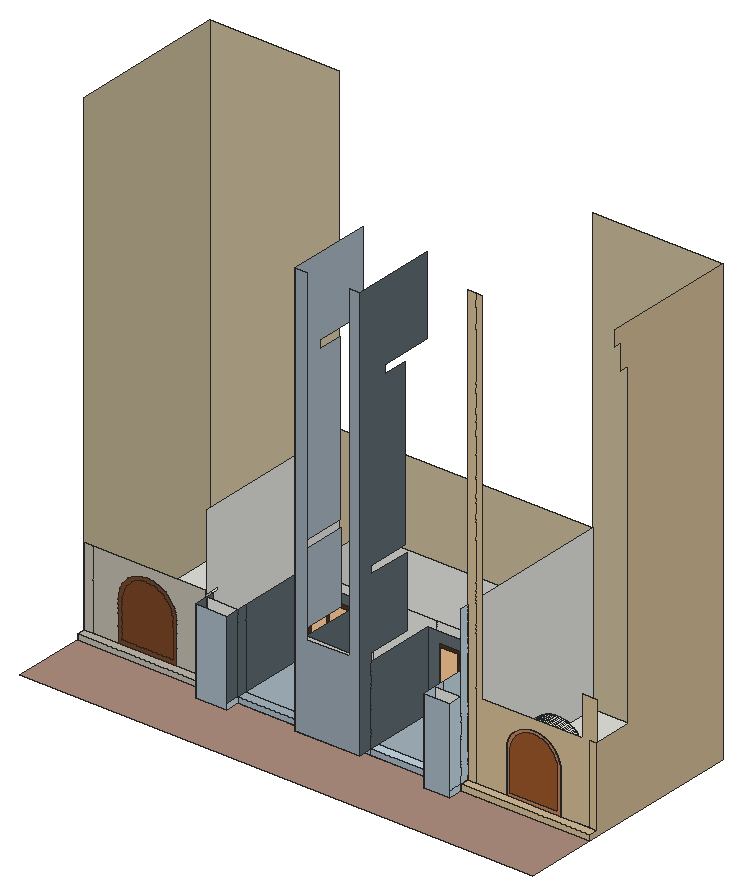
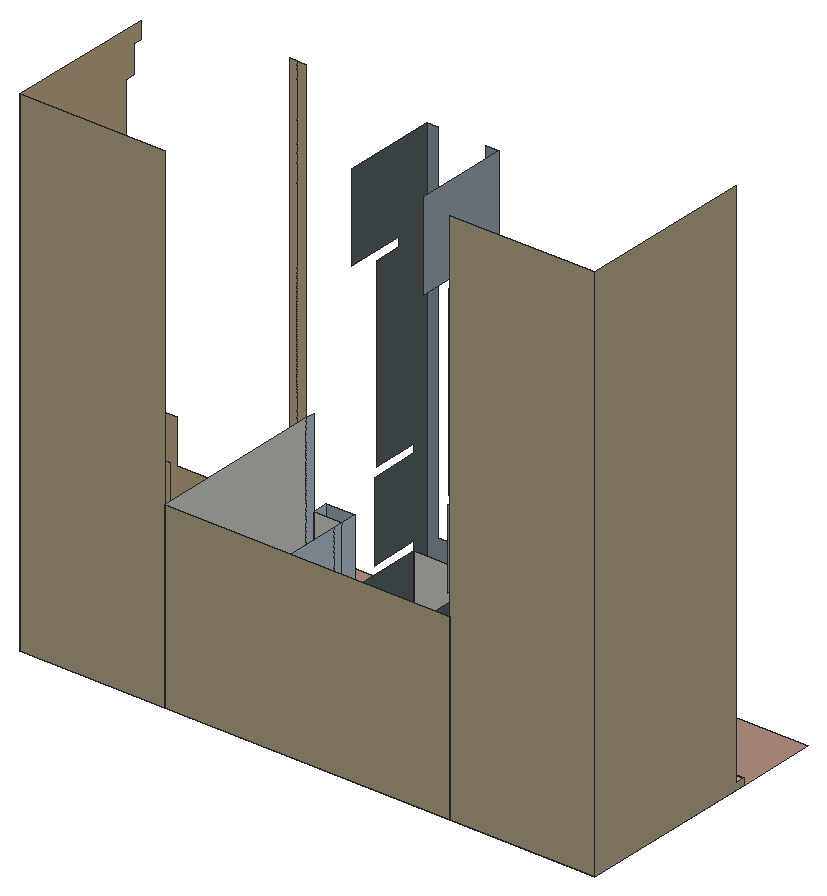
# SketchUp Ruby script. Lengths in inches.
U = 1.inch
M = Sketchup.active_model
def pt(a) = Geom::Point3d.new(a.map { |v| v * U })
def face(e, loops, mat)
  f = e.add_face(loops[0].map { |a| pt(a) })
  loops[1..].each { |l| e.add_face(l.map { |a| pt(a) }).erase! }
  f.material = f.back_material = mat if mat
  f
end
# faces: each face lists its corners as indices into pts; further lists are holes
def faces(e, pts, list, mat = nil) = list.each { |f| face(e, (f[0].is_a?(Array) ? f : [f]).map { |l| l.map { |i| pts[i] } }, mat) }
# xy, xz, yz: faces in a plane at the given z, y or x. An outline is a flat list of corners, or four numbers for a rectangle; further outlines are holes
def ring(l) = l.size == 4 ? [[l[0], l[1]], [l[2], l[1]], [l[2], l[3]], [l[0], l[3]]] : l.each_slice(2).to_a
def flat(e, list, mat, &to3) = list.each { |f| face(e, (f[0].is_a?(Array) ? f : [f]).map { |l| ring(l).map { |u, v| to3.(u, v) } }, mat) }
def xy(e, z, list, mat = nil) = flat(e, list, mat) { |x, y| [x, y, z] }
def xz(e, y, list, mat = nil) = flat(e, list, mat) { |x, z| [x, y, z] }
def yz(e, x, list, mat = nil) = flat(e, list, mat) { |y, z| [x, y, z] }
def lines(e, pts, list) = list.each { |a, b| e.add_line(pt(pts[a]), pt(pts[b])) }
# prism: a flat outline (further loops are holes) pulled along v
def prism(e, loops, v, mat = nil)
  f = face(e, loops, mat); d = Geom::Vector3d.new(v.map { |x| x * U })
  f.pushpull(f.normal.samedirection?(d) ? d.length : -d.length)
end
def box(e, o, s, mat = nil) = prism(e, [[o, [o[0] + s[0], o[1], o[2]], [o[0] + s[0], o[1] + s[1], o[2]], [o[0], o[1] + s[1], o[2]]]], [0, 0, s[2]], mat)
def at(x, y, z, deg = 0) = Geom::Transformation.translation(pt([x, y, z])) * Geom::Transformation.rotation(ORIGIN, Z_AXIS, deg.degrees)
def axes(o, x, y, z) = Geom::Transformation.new([*x, 0, *y, 0, *z, 0, *pt(o).to_a, 1])
def part(name) = M.definitions.add(name)
# library, detail: a bought-in or finely detailed component or shape, given as its bounding box
def library(name, o, s) = part(name).tap { |d| box(d.entities, o, s) }
def detail(e, o, s) = box(e.add_group.entities, o, s)
def put(e, d, t, mat = nil) = e.add_instance(d, t).tap { |i| i.material = mat if mat }
def group(e, t, mat = nil) = e.add_group.tap { |g| g.transformation = t; g.material = mat if mat }.entities
root = M.entities
M.materials.add("[Cinder Block]").color = [191, 184, 171]
M.materials.add("[Color C02]").color = [255, 204, 153]
M.materials.add("[Formica Beige]").color = [211, 187, 149]
M.materials.add("[Formica Speckled Grey]").color = [94, 105, 111]
M.materials.add("[Pavers Modular Brick]").color = [175, 143, 129]
M.materials.add("[Quartz Light Brown]").color = [199, 184, 152]
M.materials.add("[Terrazzo Light Blue]").color = [151, 165, 175]
M.materials.add("[Terrazzo Light Blue]1").color = [165, 180, 191]
M.materials.add("[Terrazzo Light Blue]2").color = [196, 214, 227]
M.materials.add("[Wood Cherry Original]").color = [152, 86, 42]
M.materials.add("[Wood Veneer 01]1").color = [81, 47, 25]
M.materials.add("[Wood Veneer 01]2").color = [120, 70, 37]
M.materials.add("[Wood Veneer 02]").color = [190, 128, 91]
xy(root,0,[[198.57,88.2,246.77,110.07],[549.2,88.2,588.3,110.07],[0,110.07,198.57,364.125],[198.57,110.07,588.3,364.125],[588.3,110.07,786.87,364.125]])
xy(root,0,[[0,0,0,110.07,198.57,110.07,198.57,88.2,246.77,88.2,246.77,110.07,549.2,110.07,549.2,88.2,588.3,88.2,588.3,110.07,786.87,110.07,786.87,0]],"[Pavers Modular Brick]")
xy(root,9,[[351.88,88.2,450.54,110.07],[648.15,122.79,731.58,168.17],[246.77,237.1,549.2,350.21]])
xy(root,9,[[0,110.07,198.57,122.79]],"[Cinder Block]")
xy(root,9,[[588.3,110.07,786.87,122.79]],"[Formica Beige]")
xy(root,9,[[246.77,110.07,351.88,123.98],[246.77,123.98,351.88,219.13],[450.54,123.98,549.2,219.13]],"[Terrazzo Light Blue]1")
xy(root,9,[[450.54,110.07,549.2,123.98]],"[Terrazzo Light Blue]2")
xz(root,88.2,[[351.88,9,450.54,9,450.54,645,435.37,645,435.37,140.5,369.87,140.5,369.87,645,351.88,645]],"[Terrazzo Light Blue]")
xz(root,88.2,[[198.57,0,246.77,129],[549.2,0,588.3,129]],"[Terrazzo Light Blue]1")
xz(root,110.07,[[198.57,0,246.77,129],[549.2,0,588.3,129],[351.88,9,450.54,129]])
xz(root,110.07,[[0,0,198.57,9]],"[Cinder Block]")
xz(root,110.07,[[588.3,0,786.87,9]],"[Formica Beige]")
xz(root,110.07,[[246.77,0,351.88,9],[351.88,0,450.54,9],[450.54,0,549.2,9]],"[Terrazzo Light Blue]1")
xz(root,122.79,[[0,9,12.72,129],[12.72,9,51.6,9,51.6,65.125,51.48,67.62,51.49,70.12,51.65,72.62,51.9375,75.1,52.36,77.5625,52.92,80,53.61,82.4,54.4375,84.76,55.39,87.07,56.46,89.33,57.66,91.52,58.98,93.64,60.41,95.69,61.96,97.66,63.6,99.54,65.35,101.33,67.2,103.01,69.13,104.6,71.15,106.07,73.24,107.43,75.41,108.68,77.64,109.8,79.93,110.8,82.28,111.68,84.66,112.42,87.09,113.03,89.54,113.51,92.02,113.85,94.51,114.06,97.01,114.125,99.5,114.06,102,113.85,104.47,113.51,106.93,113.03,109.35,112.42,111.74,111.68,114.08,110.8,116.37,109.8,118.6,108.68,120.77,107.43,122.86,106.07,124.88,104.6,126.82,103.01,128.66,101.33,130.41,99.54,132.06,97.66,133.6,95.69,135.03,93.64,136.35,91.52,137.55,89.33,138.625,87.07,139.58,84.76,140.4,82.4,141.09,80,141.65,77.5625,142.08,75.1,142.37,72.62,142.52,70.12,142.53,67.62,142.41,65.125,142.41,9,185.85,9,185.85,129,12.72,129],[185.85,9,198.57,129]],"[Cinder Block]")
xz(root,122.79,[[588.3,9,601.02,682.5],[601.02,9,648.15,9,648.15,75.375,648.42,77.4,648.8,79.41,649.27,81.39,649.84,83.35,650.5,85.29,651.25,87.18,652.1,89.04,653.04,90.86,654.06,92.62,655.17,94.34,656.36,96,657.63,97.6,658.97,99.13,660.39,100.6,661.88,102,663.43,103.32,665.05,104.57,666.73,105.74,668.46,106.82,670.24,107.82,672.07,108.73,673.9375,109.55,675.85,110.28,677.79,110.91,679.76,111.45,681.75,111.9,683.76,112.24,685.79,112.49,687.82,112.64,689.87,112.6875,691.91,112.64,693.94,112.49,695.97,112.24,697.98,111.9,699.98,111.45,701.94,110.91,703.89,110.28,705.79,109.55,707.66,108.73,709.49,107.82,711.27,106.82,713,105.74,714.68,104.57,716.3,103.32,717.85,102,719.34,100.6,720.76,99.13,722.1,97.6,723.37,96,724.5625,94.34,725.67,92.62,726.69,90.86,727.63,89.04,728.48,87.18,729.23,85.29,729.89,83.35,730.46,81.39,730.93,79.41,731.31,77.4,731.58,75.375,731.58,9,774.15,9,774.15,129,786.87,129,786.87,189,765.67,189,765.67,129,611.125,129,611.125,682.5,601.02,682.5],[774.15,9,786.87,129]],"[Formica Beige]")
xz(root,122.79,[[653.92,14.78,725.81,14.78,725.81,74.98,725.6,76.48,725.28,78.21,724.875,79.92,724.38,81.61,723.8125,83.28,723.16,84.91,722.43,86.52,721.625,88.08,720.74,89.61,719.79,91.08,718.76,92.52,717.67,93.89,716.5,95.22,715.28,96.49,714,97.69,712.66,98.83,711.26,99.91,709.82,100.91,708.33,101.85,706.79,102.71,705.21,103.49,703.6,104.2,701.96,104.83,700.28,105.38,698.58,105.84,696.87,106.23,695.13,106.52,693.38,106.74,691.625,106.87,689.87,106.91,688.11,106.87,686.35,106.74,684.6,106.52,682.87,106.23,681.15,105.84,679.45,105.38,677.78,104.83,676.13,104.2,674.52,103.49,672.94,102.71,671.41,101.85,669.91,100.91,668.47,99.91,667.07,98.83,665.73,97.69,664.45,96.49,663.23,95.22,662.07,93.89,660.97,92.52,659.94,91.08,658.99,89.61,658.11,88.08,657.3,86.52,656.57,84.91,655.92,83.28,655.35,81.61,654.86,79.92,654.45,78.21,654.13,76.48,653.92,74.98]],"[Wood Cherry Original]")
xz(root,122.79,[[[51.6,9,142.41,9,142.41,65.125,142.53,67.62,142.52,70.12,142.37,72.62,142.08,75.1,141.65,77.5625,141.09,80,140.4,82.4,139.58,84.76,138.625,87.07,137.55,89.33,136.35,91.52,135.03,93.64,133.6,95.69,132.06,97.66,130.41,99.54,128.66,101.33,126.82,103.01,124.88,104.6,122.86,106.07,120.77,107.43,118.6,108.68,116.37,109.8,114.08,110.8,111.74,111.68,109.35,112.42,106.93,113.03,104.47,113.51,102,113.85,99.5,114.06,97.01,114.125,94.51,114.06,92.02,113.85,89.54,113.51,87.09,113.03,84.66,112.42,82.28,111.68,79.93,110.8,77.64,109.8,75.41,108.68,73.24,107.43,71.15,106.07,69.13,104.6,67.2,103.01,65.35,101.33,63.6,99.54,61.96,97.66,60.41,95.69,58.98,93.64,57.66,91.52,56.46,89.33,55.39,87.07,54.4375,84.76,53.61,82.4,52.92,80,52.36,77.5625,51.9375,75.1,51.65,72.62,51.49,70.12,51.48,67.62,51.6,65.125],[57.95,15.35,57.95,65.28,57.83,67.76,57.85,69.91,57.98,72.05,58.23,74.19,58.59,76.31,59.07,78.41,59.67,80.47,60.38,82.5,61.2,84.49,62.125,86.43,63.16,88.32,64.29,90.15,65.52,91.91,66.85,93.6,68.27,95.22,69.77,96.75,71.36,98.21,73.02,99.57,74.76,100.84,76.5625,102.01,78.43,103.08,80.35,104.05,82.32,104.91,84.33,105.66,86.39,106.3,88.47,106.83,90.58,107.24,92.71,107.53,94.86,107.71,97.01,107.77,99.16,107.71,101.3,107.53,103.43,107.24,105.54,106.83,107.625,106.3,109.68,105.66,111.69,104.91,113.67,104.05,115.59,103.08,117.45,102.01,119.25,100.84,120.99,99.57,122.65,98.21,124.24,96.75,125.74,95.22,127.16,93.6,128.49,91.91,129.72,90.15,130.86,88.32,131.89,86.43,132.8125,84.49,133.63,82.5,134.34,80.47,134.9375,78.41,135.42,76.31,135.78,74.19,136.03,72.05,136.16,69.91,136.18,67.76,136.06,65.28,136.06,15.35]],[57.95,15.35,136.06,15.35,136.06,65.28,136.18,67.76,136.16,69.91,136.03,72.05,135.78,74.19,135.42,76.31,134.9375,78.41,134.34,80.47,133.63,82.5,132.8125,84.49,131.89,86.43,130.86,88.32,129.72,90.15,128.49,91.91,127.16,93.6,125.74,95.22,124.24,96.75,122.65,98.21,120.99,99.57,119.25,100.84,117.45,102.01,115.59,103.08,113.67,104.05,111.69,104.91,109.68,105.66,107.625,106.3,105.54,106.83,103.43,107.24,101.3,107.53,99.16,107.71,97.01,107.77,94.86,107.71,92.71,107.53,90.58,107.24,88.47,106.83,86.39,106.3,84.33,105.66,82.32,104.91,80.35,104.05,78.43,103.08,76.5625,102.01,74.76,100.84,73.02,99.57,71.36,98.21,69.77,96.75,68.27,95.22,66.85,93.6,65.52,91.91,64.29,90.15,63.16,88.32,62.125,86.43,61.2,84.49,60.38,82.5,59.67,80.47,59.07,78.41,58.59,76.31,58.23,74.19,57.98,72.05,57.85,69.91,57.83,67.76,57.95,65.28]],"[Wood Veneer 01]2")
xz(root,122.79,[[[648.15,9,731.58,9,731.58,75.375,731.31,77.4,730.93,79.41,730.46,81.39,729.89,83.35,729.23,85.29,728.48,87.18,727.63,89.04,726.69,90.86,725.67,92.62,724.5625,94.34,723.37,96,722.1,97.6,720.76,99.13,719.34,100.6,717.85,102,716.3,103.32,714.68,104.57,713,105.74,711.27,106.82,709.49,107.82,707.66,108.73,705.79,109.55,703.89,110.28,701.94,110.91,699.98,111.45,697.98,111.9,695.97,112.24,693.94,112.49,691.91,112.64,689.87,112.6875,687.82,112.64,685.79,112.49,683.76,112.24,681.75,111.9,679.76,111.45,677.79,110.91,675.85,110.28,673.9375,109.55,672.07,108.73,670.24,107.82,668.46,106.82,666.73,105.74,665.05,104.57,663.43,103.32,661.88,102,660.39,100.6,658.97,99.13,657.63,97.6,656.36,96,655.17,94.34,654.06,92.62,653.04,90.86,652.1,89.04,651.25,87.18,650.5,85.29,649.84,83.35,649.27,81.39,648.8,79.41,648.42,77.4,648.15,75.375],[653.92,14.78,653.92,74.98,654.13,76.48,654.45,78.21,654.86,79.92,655.35,81.61,655.92,83.28,656.57,84.91,657.3,86.52,658.11,88.08,658.99,89.61,659.94,91.08,660.97,92.52,662.07,93.89,663.23,95.22,664.45,96.49,665.73,97.69,667.07,98.83,668.47,99.91,669.91,100.91,671.41,101.85,672.94,102.71,674.52,103.49,676.13,104.2,677.78,104.83,679.45,105.38,681.15,105.84,682.87,106.23,684.6,106.52,686.35,106.74,688.11,106.87,689.87,106.91,691.625,106.87,693.38,106.74,695.13,106.52,696.87,106.23,698.58,105.84,700.28,105.38,701.96,104.83,703.6,104.2,705.21,103.49,706.79,102.71,708.33,101.85,709.82,100.91,711.26,99.91,712.66,98.83,714,97.69,715.28,96.49,716.5,95.22,717.67,93.89,718.76,92.52,719.79,91.08,720.74,89.61,721.625,88.08,722.43,86.52,723.16,84.91,723.8125,83.28,724.38,81.61,724.875,79.92,725.28,78.21,725.6,76.48,725.81,74.98,725.81,14.78]]],"[Wood Veneer 02]")
xz(root,168.17,[[[648.15,9,731.58,9,731.58,75.375,731.31,77.4,730.93,79.41,730.46,81.39,729.89,83.35,729.23,85.29,728.48,87.18,727.63,89.04,726.69,90.86,725.67,92.62,724.5625,94.34,723.37,96,722.1,97.6,720.76,99.13,719.34,100.6,717.85,102,716.3,103.32,714.68,104.57,713,105.74,711.27,106.82,709.49,107.82,707.66,108.73,705.79,109.55,703.89,110.28,701.94,110.91,699.98,111.45,697.98,111.9,695.97,112.24,693.94,112.49,691.91,112.64,689.87,112.6875,687.82,112.64,685.79,112.49,683.76,112.24,681.75,111.9,679.76,111.45,677.79,110.91,675.85,110.28,673.9375,109.55,672.07,108.73,670.24,107.82,668.46,106.82,666.73,105.74,665.05,104.57,663.43,103.32,661.88,102,660.39,100.6,658.97,99.13,657.63,97.6,656.36,96,655.17,94.34,654.06,92.62,653.04,90.86,652.1,89.04,651.25,87.18,650.5,85.29,649.84,83.35,649.27,81.39,648.8,79.41,648.42,77.4,648.15,75.375],[652.4375,13.29,652.4375,75.08,652.66,76.71,653,78.52,653.42,80.3,653.93,82.0625,654.52,83.8,655.2,85.5,655.96,87.17,656.8,88.8,657.72,90.38,658.72,91.92,659.78,93.41,660.92,94.85,662.13,96.23,663.4,97.54,664.74,98.8,666.14,99.99,667.59,101.11,669.09,102.15,670.65,103.13,672.25,104.02,673.89,104.84,675.57,105.58,677.28,106.23,679.02,106.8,680.79,107.29,682.58,107.68,684.38,108,686.2,108.22,688.03,108.35,689.87,108.4,691.7,108.35,693.53,108.22,695.35,108,697.15,107.68,698.94,107.29,700.71,106.8,702.45,106.23,704.16,105.58,705.84,104.84,707.48,104.02,709.08,103.13,710.64,102.15,712.14,101.11,713.59,99.99,714.99,98.8,716.33,97.54,717.6,96.23,718.81,94.85,719.95,93.41,721.02,91.92,722.01,90.38,722.93,88.8,723.77,87.17,724.53,85.5,725.21,83.8,725.8,82.0625,726.3125,80.3,726.74,78.52,727.07,76.71,727.29,75.08,727.29,13.29]],[652.4375,13.29,727.29,13.29,727.29,75.08,727.07,76.71,726.74,78.52,726.3125,80.3,725.8,82.0625,725.21,83.8,724.53,85.5,723.77,87.17,722.93,88.8,722.01,90.38,721.02,91.92,719.95,93.41,718.81,94.85,717.6,96.23,716.33,97.54,714.99,98.8,713.59,99.99,712.14,101.11,710.64,102.15,709.08,103.13,707.48,104.02,705.84,104.84,704.16,105.58,702.45,106.23,700.71,106.8,698.94,107.29,697.15,107.68,695.35,108,693.53,108.22,691.7,108.35,689.87,108.4,688.03,108.35,686.2,108.22,684.38,108,682.58,107.68,680.79,107.29,679.02,106.8,677.28,106.23,675.57,105.58,673.89,104.84,672.25,104.02,670.65,103.13,669.09,102.15,667.59,101.11,666.14,99.99,664.74,98.8,663.4,97.54,662.13,96.23,660.92,94.85,659.78,93.41,658.72,91.92,657.72,90.38,656.8,88.8,655.96,87.17,655.2,85.5,654.52,83.8,653.93,82.0625,653.42,80.3,653,78.52,652.66,76.71,652.4375,75.08]])
xz(root,219.13,[[270.19,12.94,293.73,108.04],[298.46,12.94,325.93,108.04],[471.125,13.31,495.12,107.5],[500.07,13.31,525.26,107.5]],"[Color C02]")
xz(root,219.13,[[246.77,9,265.64,9,265.64,114.1,330.47,114.1,330.47,9,351.88,9,351.88,129,246.77,129],[450.54,9,467.28,9,467.28,112.63,529.11,112.63,529.11,9,549.2,9,549.2,129,450.54,129]],"[Formica Speckled Grey]")
xz(root,219.13,[[265.64,9,330.47,12.94],[467.28,9,529.11,13.31],[265.64,12.94,270.19,12.94,270.19,108.04,325.93,108.04,325.93,12.94,330.47,12.94,330.47,114.1,265.64,114.1],[293.73,12.94,298.46,108.04],[467.28,13.31,471.125,13.31,471.125,107.5,525.26,107.5,525.26,13.31,529.11,13.31,529.11,112.63,467.28,112.63],
  [495.12,13.31,500.07,107.5]],"[Wood Veneer 01]1")
xz(root,237.1,[[246.77,9,351.88,129],[351.88,9,450.54,129],[450.54,9,549.2,129]])
xz(root,350.21,[[246.77,9,549.2,129]])
xz(root,364.125,[[0,0,198.57,740.5625],[198.57,0,588.3,249],[588.3,0,786.87,682.5]],"[Quartz Light Brown]")
yz(root,0,[[110.07,0,110.07,9,122.79,9,122.79,740.5625,364.125,740.5625,364.125,0]],"[Quartz Light Brown]")
yz(root,198.57,[[110.07,0,110.07,9,122.79,9,122.79,129,131.79,129,131.79,133.5625,110.07,133.5625,110.07,249,364.125,249,364.125,0]])
yz(root,198.57,[[88.2,0,110.07,9],[88.2,9,110.07,129],[110.07,9,122.79,129]],"[Formica Speckled Grey]")
yz(root,246.77,[[237.1,9,350.21,129]])
yz(root,246.77,[[88.2,9,110.07,129],[110.07,9,123.98,129],[123.98,9,219.13,129]],"[Formica Speckled Grey]")
yz(root,246.77,[[88.2,0,110.07,9]],"[Terrazzo Light Blue]2")
yz(root,351.88,[[110.07,9,219.13,129]],"[Formica Speckled Grey]")
yz(root,351.88,[[88.2,9,88.2,645,216.84,645,216.84,525,135.71,525,135.71,513,174.4375,513,174.4375,261,110.07,261,110.07,249,175.78,249,175.78,141,110.07,141,110.07,9]],"[Terrazzo Light Blue]1")
yz(root,450.54,[[88.2,9,110.07,9,110.07,141,177.84,141,177.84,249,110.07,249,110.07,261,174.4375,261,174.4375,513,135.71,513,135.71,525,216.84,525,216.84,645,88.2,645],[110.07,9,219.13,129]],"[Formica Speckled Grey]")
yz(root,549.2,[[237.1,9,350.21,129]])
yz(root,549.2,[[88.2,0,110.07,9],[88.2,9,110.07,129],[110.07,9,123.98,129],[123.98,9,219.13,129]],"[Terrazzo Light Blue]2")
yz(root,588.3,[[110.07,0,364.125,0,364.125,249,122.79,249,122.79,9,110.07,9]])
yz(root,588.3,[[88.2,0,110.07,9],[88.2,9,110.07,129],[110.07,9,122.79,249]],"[Terrazzo Light Blue]2")
yz(root,648.15,[[122.79,9,168.17,75.375]])
yz(root,731.58,[[122.79,9,168.17,75.375]])
yz(root,786.87,[[110.07,0,364.125,0,364.125,682.5,157.7,682.5,157.7,658.875,169.39,658.875,169.39,621,182.57,621,182.57,129,122.79,129,122.79,9,110.07,9]],"[Formica Beige]")
p = [[648.15,168.17,75.375],[648.42,168.17,77.4],[648.42,122.79,77.4],[648.15,122.79,75.375],[731.31,168.17,77.4],[731.58,168.17,75.375],
  [731.58,122.79,75.375],[731.31,122.79,77.4],[648.8,168.17,79.41],[648.8,122.79,79.41],[730.93,168.17,79.41],[730.93,122.79,79.41],
  [649.27,168.17,81.39],[649.27,122.79,81.39],[730.46,168.17,81.39],[730.46,122.79,81.39],[649.84,168.17,83.35],[649.84,122.79,83.35],
  [729.89,168.17,83.35],[729.89,122.79,83.35],[650.5,168.17,85.29],[650.5,122.79,85.29],[729.23,168.17,85.29],[729.23,122.79,85.29],
  [651.25,168.17,87.18],[651.25,122.79,87.18],[728.48,168.17,87.18],[728.48,122.79,87.18],[652.1,168.17,89.04],[652.1,122.79,89.04],
  [727.63,168.17,89.04],[727.63,122.79,89.04],[653.04,168.17,90.86],[653.04,122.79,90.86],[726.69,168.17,90.86],[726.69,122.79,90.86],
  [654.06,168.17,92.62],[654.06,122.79,92.62],[725.67,168.17,92.62],[725.67,122.79,92.62],[655.17,168.17,94.34],[655.17,122.79,94.34],
  [724.5625,168.17,94.34],[724.5625,122.79,94.34],[656.36,168.17,96],[656.36,122.79,96],[723.37,168.17,96],[723.37,122.79,96],
  [657.63,168.17,97.6],[657.63,122.79,97.6],[722.1,168.17,97.6],[722.1,122.79,97.6],[658.97,168.17,99.13],[658.97,122.79,99.13],
  [720.76,168.17,99.13],[720.76,122.79,99.13],[660.39,168.17,100.6],[660.39,122.79,100.6],[719.34,168.17,100.6],[719.34,122.79,100.6],
  [661.88,168.17,102],[661.88,122.79,102],[717.85,168.17,102],[717.85,122.79,102],[663.43,168.17,103.32],[663.43,122.79,103.32],
  [716.3,168.17,103.32],[716.3,122.79,103.32],[665.05,168.17,104.57],[665.05,122.79,104.57],[714.68,168.17,104.57],[714.68,122.79,104.57],
  [666.73,168.17,105.74],[666.73,122.79,105.74],[713,168.17,105.74],[713,122.79,105.74],[668.46,168.17,106.82],[668.46,122.79,106.82],
  [711.27,168.17,106.82],[711.27,122.79,106.82],[670.24,168.17,107.82],[670.24,122.79,107.82],[709.49,168.17,107.82],[709.49,122.79,107.82],
  [672.07,168.17,108.73],[672.07,122.79,108.73],[707.66,168.17,108.73],[707.66,122.79,108.73],[673.9375,168.17,109.55],[673.9375,122.79,109.55],
  [705.79,168.17,109.55],[705.79,122.79,109.55],[675.85,168.17,110.28],[675.85,122.79,110.28],[703.89,168.17,110.28],[703.89,122.79,110.28],
  [677.79,168.17,110.91],[677.79,122.79,110.91],[701.94,168.17,110.91],[701.94,122.79,110.91],[679.76,168.17,111.45],[679.76,122.79,111.45],
  [699.98,168.17,111.45],[699.98,122.79,111.45],[681.75,168.17,111.9],[681.75,122.79,111.9],[697.98,168.17,111.9],[697.98,122.79,111.9],
  [683.76,168.17,112.24],[683.76,122.79,112.24],[695.97,168.17,112.24],[695.97,122.79,112.24],[685.79,168.17,112.49],[685.79,122.79,112.49],
  [693.94,168.17,112.49],[693.94,122.79,112.49],[687.82,168.17,112.64],[687.82,122.79,112.64],[691.91,168.17,112.64],[691.91,122.79,112.64],
  [689.87,168.17,112.6875],[689.87,122.79,112.6875]]
faces(root,p,[[0,1,2,3],[4,5,6,7],[1,8,9,2],[10,4,7,11],[8,12,13,9],[14,10,11,15],[12,16,17,13],[18,14,15,19],
  [16,20,21,17],[22,18,19,23],[20,24,25,21],[26,22,23,27],[24,28,29,25],[30,26,27,31],[28,32,33,29],[34,30,31,35],
  [32,36,37,33],[38,34,35,39],[36,40,41,37],[42,38,39,43],[40,44,45,41],[46,42,43,47],[44,48,49,45],[50,46,47,51],
  [48,52,53,49],[54,50,51,55],[52,56,57,53],[58,54,55,59],[56,60,61,57],[62,58,59,63],[60,64,65,61],[66,62,63,67],
  [64,68,69,65],[70,66,67,71],[68,72,73,69],[74,70,71,75],[72,76,77,73],[78,74,75,79],[76,80,81,77],[82,78,79,83],
  [80,84,85,81],[86,82,83,87],[84,88,89,85],[90,86,87,91],[88,92,93,89],[94,90,91,95],[92,96,97,93],[98,94,95,99],
  [96,100,101,97],[102,98,99,103],[100,104,105,101],[106,102,103,107],[104,108,109,105],[110,106,107,111],[108,112,113,109],[114,110,111,115],
  [112,116,117,113],[118,114,115,119],[116,120,121,117],[120,118,119,121]])
